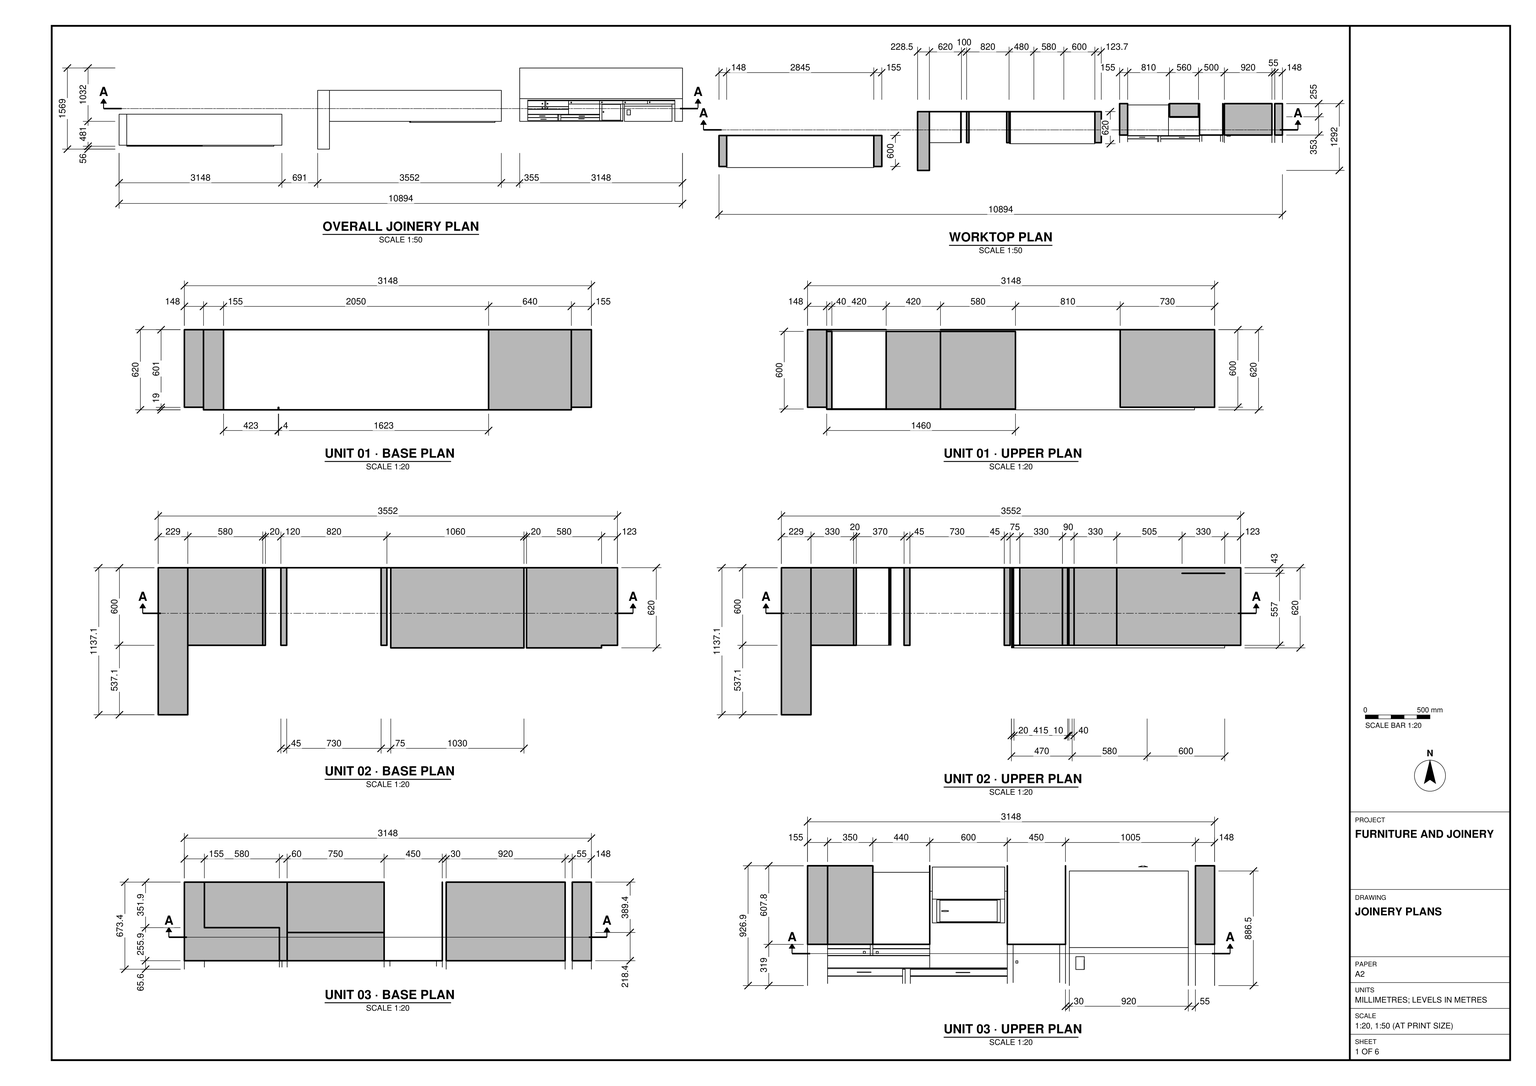
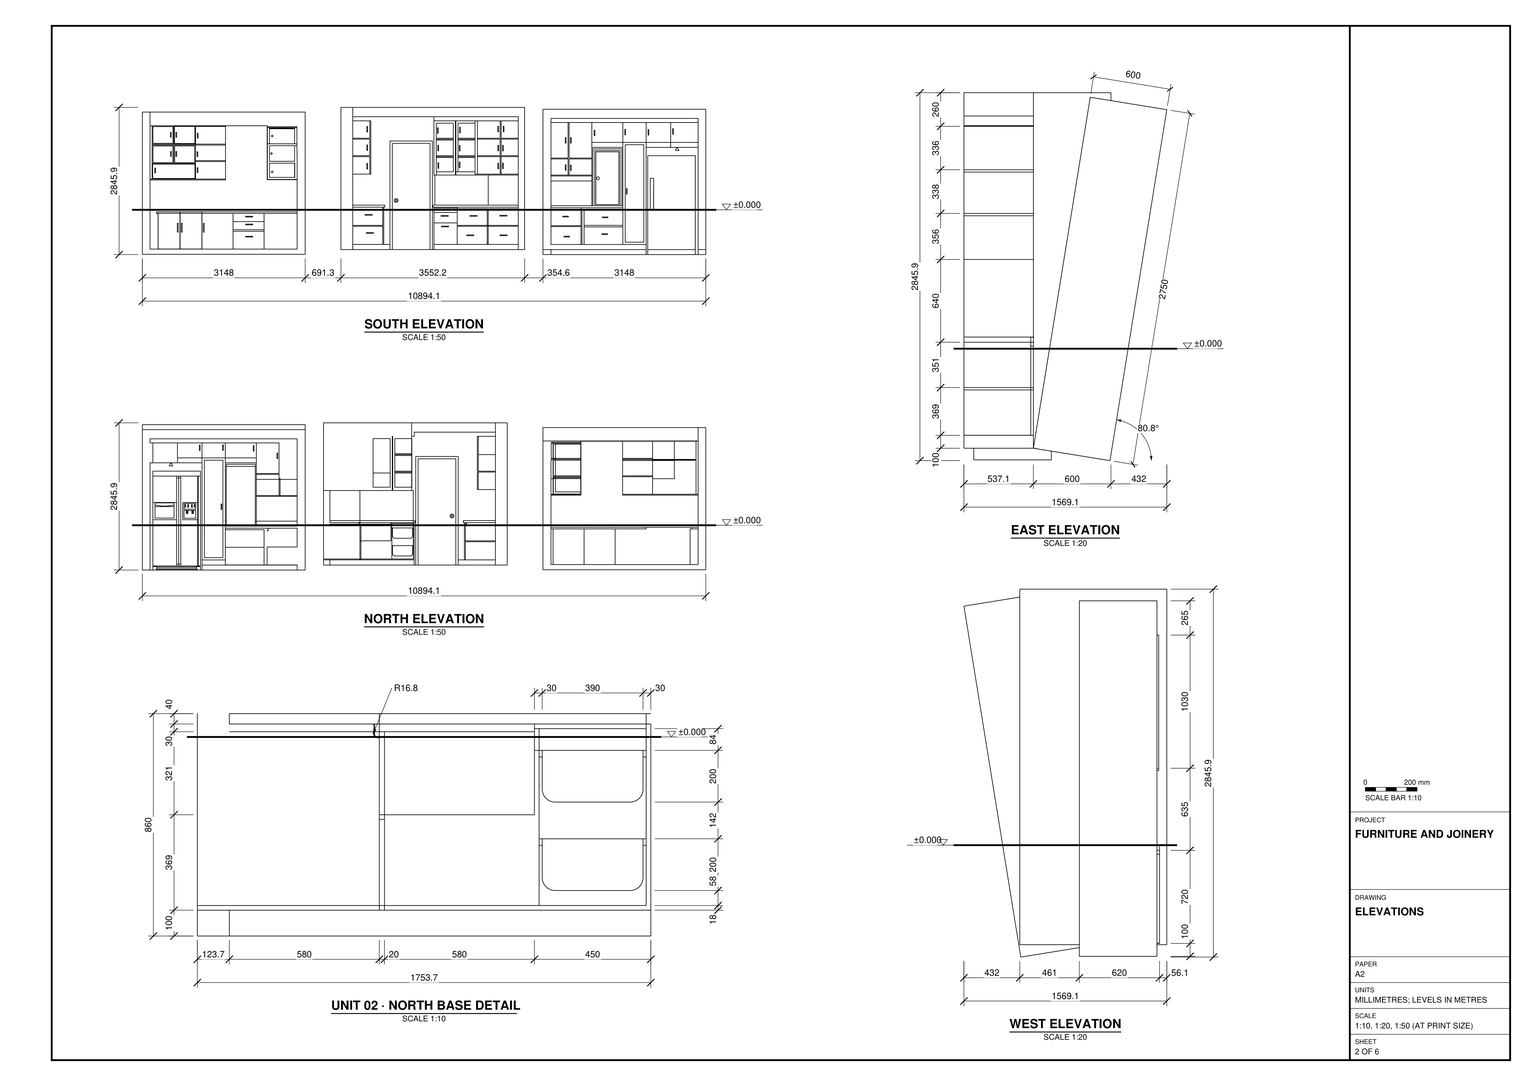
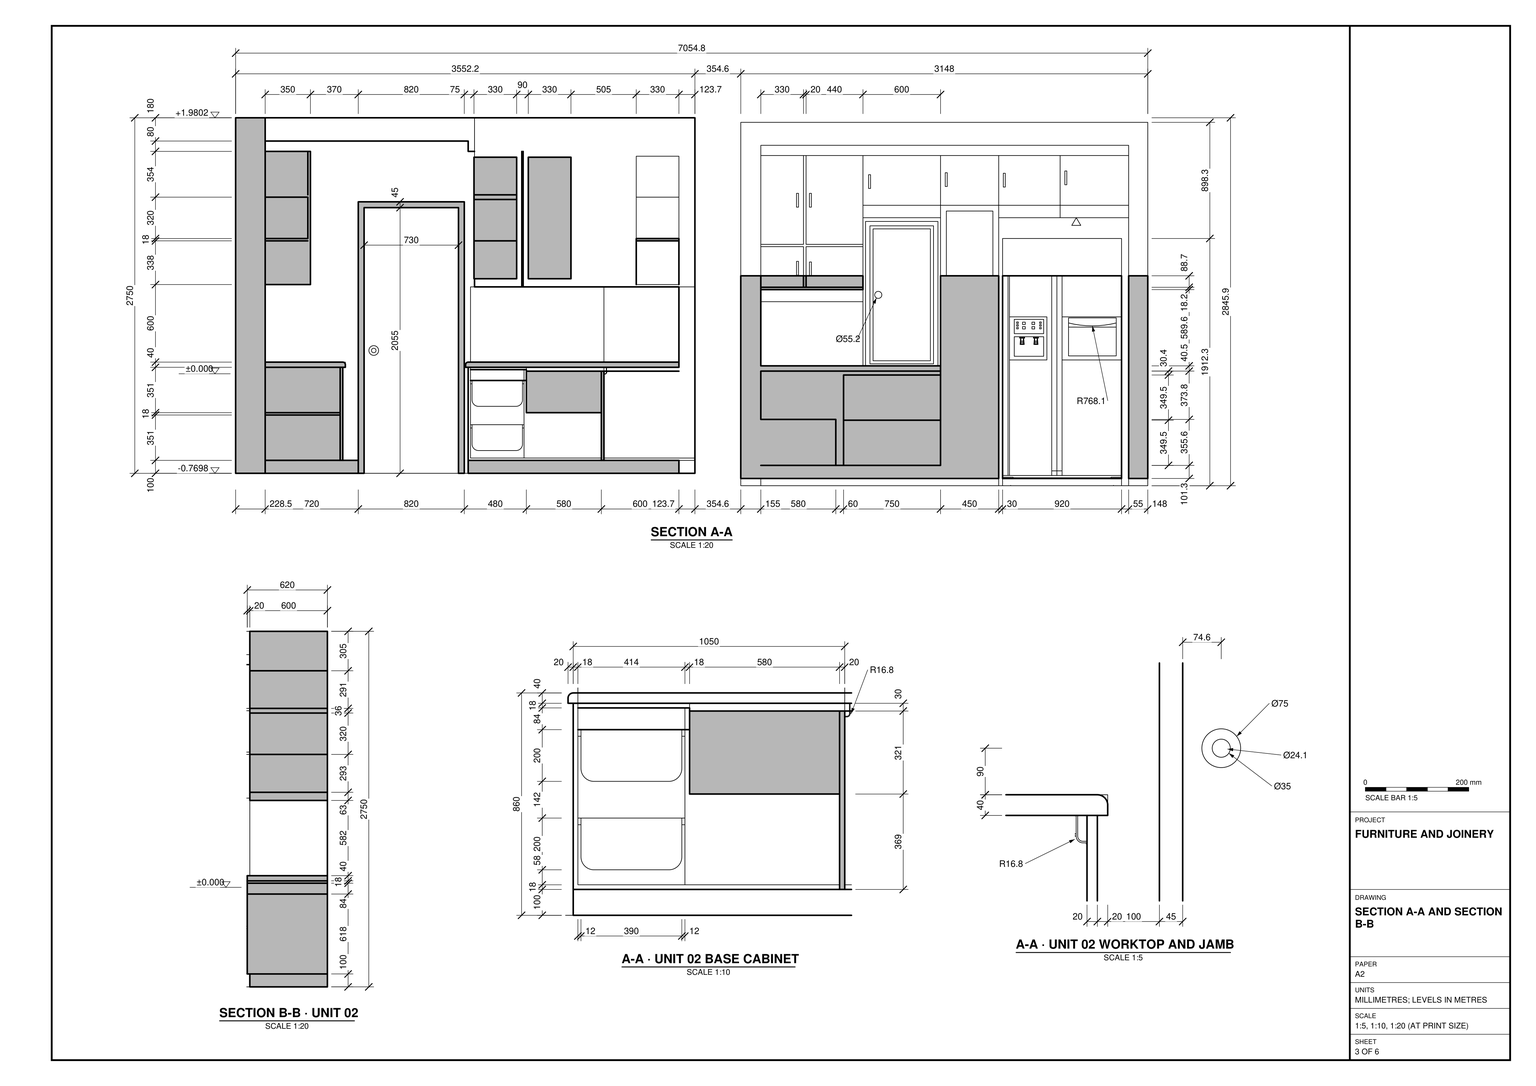
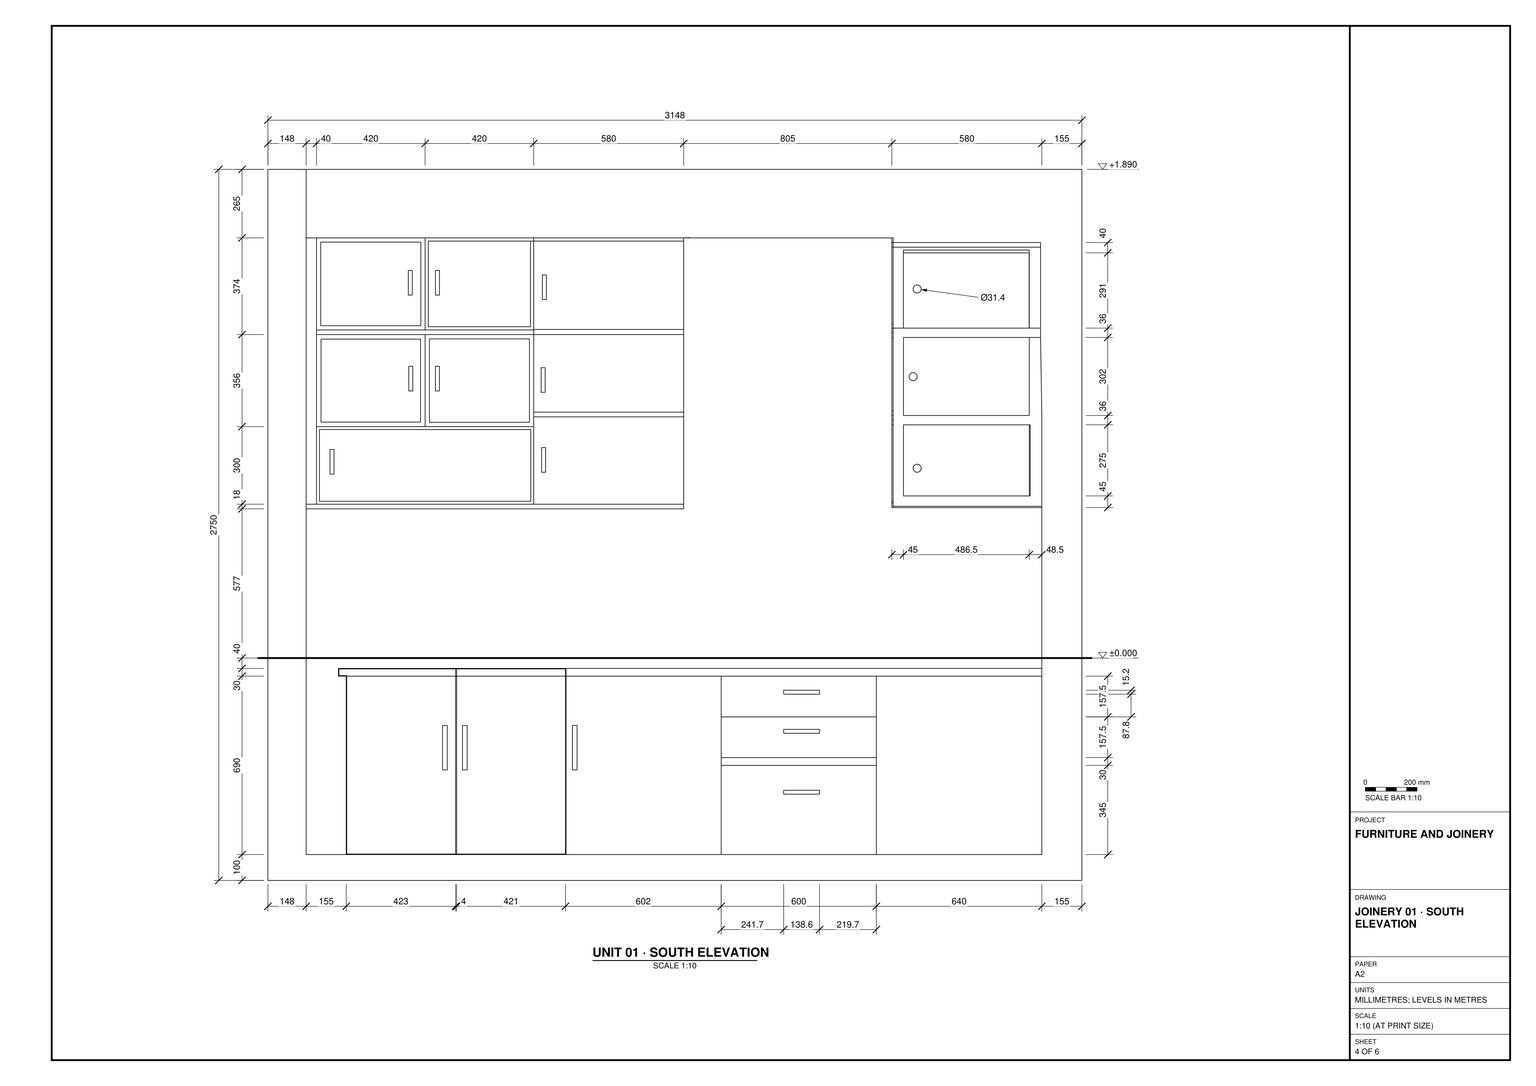
Build the three kitchen joinery runs in SketchUp from task_files/diagram_01.pdf. Work in millimetres. The complete arrangement is 10894.1 mm long, 1569.1 mm deep and 2845.9 mm high. Use the 0 mm reference level marked in the elevations; it crosses the joinery near the worktops, not at the plinths.

Use the overall plan to set out the gaps and front-to-back offsets between runs. Reading the south elevation from left to right, model the first run with base cupboards, drawers and two banks of upper cabinets separated by an open space. In the middle run, form the projecting end return and framed doorway, with worktops and storage to either side. Use the sections to model the plinths, worktop edges, shelves and stacked pull-outs at their drawn thicknesses. In the right-hand run, fit the base drawers, tall cabinet, refrigerator bay and overhead cupboards within the surround. Match the inclined and upright profiles shown together in the end elevations.

Appliances and any decorative or loose items shown may be suitable library components placed in the indicated positions. Keep each joinery assembly as a separate group or component and use components for repeated parts. Save one SketchUp model as output_files/three_kitchen_joinery_runs.skp.

# SketchUp Ruby script. Lengths in millimetres.
U = 1.mm
M = Sketchup.active_model
def pt(a) = Geom::Point3d.new(a.map { |v| v * U })
def face(e, loops, mat)
  f = e.add_face(loops[0].map { |a| pt(a) })
  loops[1..].each { |l| e.add_face(l.map { |a| pt(a) }).erase! }
  f.material = f.back_material = mat if mat
  f
end
# faces: each face lists its corners as indices into pts; further lists are holes
def faces(e, pts, list, mat = nil) = list.each { |f| face(e, (f[0].is_a?(Array) ? f : [f]).map { |l| l.map { |i| pts[i] } }, mat) }
# xy, xz, yz: faces in a plane at the given z, y or x. An outline is a flat list of corners, or four numbers for a rectangle; further outlines are holes
def ring(l) = l.size == 4 ? [[l[0], l[1]], [l[2], l[1]], [l[2], l[3]], [l[0], l[3]]] : l.each_slice(2).to_a
def flat(e, list, mat, &to3) = list.each { |f| face(e, (f[0].is_a?(Array) ? f : [f]).map { |l| ring(l).map { |u, v| to3.(u, v) } }, mat) }
def xy(e, z, list, mat = nil) = flat(e, list, mat) { |x, y| [x, y, z] }
def xz(e, y, list, mat = nil) = flat(e, list, mat) { |x, z| [x, y, z] }
def yz(e, x, list, mat = nil) = flat(e, list, mat) { |y, z| [x, y, z] }
def lines(e, pts, list) = list.each { |a, b| e.add_line(pt(pts[a]), pt(pts[b])) }
# prism: a flat outline (further loops are holes) pulled along v
def prism(e, loops, v, mat = nil)
  f = face(e, loops, mat); d = Geom::Vector3d.new(v.map { |x| x * U })
  f.pushpull(f.normal.samedirection?(d) ? d.length : -d.length)
end
def box(e, o, s, mat = nil) = prism(e, [[o, [o[0] + s[0], o[1], o[2]], [o[0] + s[0], o[1] + s[1], o[2]], [o[0], o[1] + s[1], o[2]]]], [0, 0, s[2]], mat)
def at(x, y, z, deg = 0) = Geom::Transformation.translation(pt([x, y, z])) * Geom::Transformation.rotation(ORIGIN, Z_AXIS, deg.degrees)
def axes(o, x, y, z) = Geom::Transformation.new([*x, 0, *y, 0, *z, 0, *pt(o).to_a, 1])
def part(name) = M.definitions.add(name)
# library, detail: a bought-in or finely detailed component or shape, given as its bounding box
def library(name, o, s) = part(name).tap { |d| box(d.entities, o, s) }
def detail(e, o, s) = box(e.add_group.entities, o, s)
def put(e, d, t, mat = nil) = e.add_instance(d, t).tap { |i| i.material = mat if mat }
def group(e, t, mat = nil) = e.add_group.tap { |g| g.transformation = t; g.material = mat if mat }.entities
root = M.entities
M.materials.add("A02_Rose_Quartz").color = [255, 153, 153]
M.materials.add("Asphalt_06_1K").color = [164, 157, 139]
M.materials.add("Denim_03_1K").color = [93, 106, 119]
M.materials.add("Glass_Basic_01").color = [161, 173, 186]
M.materials["Glass_Basic_01"].alpha = 0.2
M.materials.add("Glass_Safety_01").color = [204, 235, 244]
M.materials["Glass_Safety_01"].alpha = 0.2
M.materials.add("M09_Shadow_Night").color = [0, 0, 0]
M.materials.add("Wood_Floor_12_1K").color = [92, 75, 65]
M.materials.add("Wood_Veneer_15_1K").color = [103, 69, 45]
M.materials.add("glass").color = [0, 0, 0]
M.materials.add("white").color = [0, 0, 0]
c1 = library("fgkjh",[-49,-117.2,0],[98,234.4,0.1])
c2 = library("fkgjdg",[-460,-920,0],[920,1840,0.1])
c3 = part("sgdg")
p = [[83.1,0,0],[-83.1,-96,0],[-83.1,96,0]]
lines(c3.entities,p,[[0,1],[1,2],[2,0]])
c4 = library("Group\#26",[0,0,0],[920,1840,600])
c5 = part("fgklj")
p = [[-145,-100,0],[145,-100,0],[148.3,-99.9,0],[151.5,-99.6,0],[154.8,-99,0],[157.9,-98.3,0],
  [161.1,-97.3,0],[164.1,-96.2,0],[167.1,-94.8,0],[170,-93.3,0],[172.8,-91.6,0],[175.4,-89.7,0],
  [178,-87.6,0],[180.4,-85.4,0],[182.6,-83,0],[184.7,-80.4,0],[186.6,-77.8,0],[188.3,-75,0],
  [189.8,-72.1,0],[191.2,-69.1,0],[192.3,-66.1,0],[193.3,-62.9,0],[194,-59.8,0],[194.6,-56.5,0],
  [194.9,-53.3,0],[195,-50,0],[195,100,0],[-195,100,0],[-195,-50,0],[-194.9,-53.3,0],
  [-194.6,-56.5,0],[-194,-59.8,0],[-193.3,-62.9,0],[-192.3,-66.1,0],[-191.2,-69.1,0],[-189.8,-72.1,0],
  [-188.3,-75,0],[-186.6,-77.8,0],[-184.7,-80.4,0],[-182.6,-83,0],[-180.4,-85.4,0],[-178,-87.6,0],
  [-175.4,-89.7,0],[-172.8,-91.6,0],[-170,-93.3,0],[-167.1,-94.8,0],[-164.1,-96.2,0],[-161.1,-97.3,0],
  [-157.9,-98.3,0],[-154.8,-99,0],[-151.5,-99.6,0],[-148.3,-99.9,0],[-207,100,0],[-207,74.5,0],
  [-195,74.5,0],[207,100,0],[207,74.5,0],[195,74.5,0]]
lines(c5.entities,p,[[0,1],[1,2],[2,3],[3,4],[4,5],[5,6],[6,7],[7,8],[8,9],[9,10],[10,11],[11,12],
  [12,13],[13,14],[14,15],[15,16],[16,17],[17,18],[18,19],[19,20],[20,21],[21,22],[22,23],[23,24],
  [24,25],[25,26],[26,27],[27,28],[28,29],[29,30],[30,31],[31,32],[32,33],[33,34],[34,35],[35,36],
  [36,37],[37,38],[38,39],[39,40],[40,41],[41,42],[42,43],[43,44],[44,45],[45,46],[46,47],[47,48],
  [48,49],[49,50],[50,51],[51,0],[27,52],[52,53],[53,54],[54,27],[26,55],[55,56],[56,57],[57,26]])
g1 = group(root,at(7746.2,1129.4,-350.7))
yz(g1,0,[[0,0,-592.3,95.9,-152.6,2810.6,439.7,2714.6]])
yz(g1,155,[[72.1,445.2,75,463,-517.3,558.9,-520.2,541.1],[137.5,848.9,230.5,1423.5,-361.7,1519.4,-454.8,944.9]])
yz(g1,155,[[75,463,-517.3,558.9,-461.2,905.4,131.1,809.5],[230.5,1423.5,-361.7,1519.4,-358.9,1537.1,233.4,1441.2],[233.4,1441.2,-358.9,1537.1,-308.3,1849.1,283.9,1753.2],[283.9,1753.2,-308.3,1849.1,-305.5,1866.9,286.8,1770.9],[286.8,1770.9,-305.5,1866.9,-194.2,2553.9,398.1,2458],
  [398.1,2458,-194.2,2553.9,-181.4,2632.9,410.9,2536.9]],"Wood_Floor_12_1K")
yz(g1,485,[[233.4,1441.2,283.9,1753.2,-308.3,1849.1,-358.9,1537.1]])
yz(g1,505,[[233.4,1441.2,283.9,1753.2,-308.3,1849.1,-358.9,1537.1],[286.8,1770.9,398.1,2458,-194.2,2553.9,-305.5,1866.9]])
yz(g1,735,[[16,98.7,-576.3,194.6,-520.2,541.1,72.1,445.2]])
yz(g1,795,[[16,98.7,71.1,439.3,-521.1,535.2,-576.3,194.6],[71.1,439.3,75.9,468.9,-516.3,564.8,-521.1,535.2],[75.9,468.9,126.3,779.8,-466,875.8,-516.3,564.8]])
yz(g1,945,[[230.5,1423.5,-361.7,1519.4,-358.9,1537.1,233.4,1441.2],[233.4,1441.2,283.9,1753.2,-308.3,1849.1,-358.9,1537.1],[283.9,1753.2,286.8,1770.9,-305.5,1866.9,-308.3,1849.1],[286.8,1770.9,-305.5,1866.9,-256.5,2168.9,335.8,2073]],"Wood_Floor_12_1K")
yz(g1,965,[[140.7,868.7,-107.4,908.9,76.5,2044.1,324.6,2003.9]])
yz(g1,1525,[[140.7,868.7,324.6,2003.9,76.5,2044.1,-107.4,908.9]])
yz(g1,1545,[[16,98.7,71.1,439.3,-521.1,535.2,-576.3,194.6],[71.1,439.3,75.9,468.9,-516.3,564.8,-521.1,535.2],[75.9,468.9,126.3,779.8,-466,875.8,-516.3,564.8],[126.3,779.8,131.1,809.5,-461.2,905.4,-466,875.8],[131.1,809.5,137.5,848.9,-454.8,944.9,-461.2,905.4]])
yz(g1,1545,[[137.5,848.9,-454.8,944.9,-256.5,2168.9,335.8,2073]],"Wood_Floor_12_1K")
yz(g1,1995,[[0,0,16,98.7,-576.3,194.6,-592.3,95.9],[16,98.7,335.8,2073,-256.5,2168.9,-576.3,194.6]],"Wood_Floor_12_1K")
yz(g1,3000,[[0,0,-592.3,95.9,-256.5,2168.9,335.8,2073],[398.1,2458,410.9,2536.9,-181.4,2632.9,-194.2,2553.9]],"Wood_Floor_12_1K")
yz(g1,3148,[[0,0,439.7,2714.6,-152.6,2810.6,-592.3,95.9]])
# 9 loose lines left out
p = [[0,0,0],[155,0,0],[155,-592.3,95.9],[0,-592.3,95.9],[1995,0,0],[1995,-592.3,95.9],
  [3000,0,0],[3148,0,0],[3148,-592.3,95.9],[3000,-592.3,95.9],[3000,398.1,2458],[2945,398.1,2458],
  [2945,335.8,2073],[3000,335.8,2073],[3148,439.7,2714.6],[0,439.7,2714.6],[155,16,98.7],[735,16,98.7],
  [735,72.1,445.2],[155,72.1,445.2],[155,75,463],[155,131.1,809.5],[735,131.1,809.5],[1545,131.1,809.5],
  [1545,137.5,848.9],[945,137.5,848.9],[155,137.5,848.9],[155,230.5,1423.5],[155,233.4,1441.2],[155,283.9,1753.2],
  [155,286.8,1770.9],[155,398.1,2458],[155,410.9,2536.9],[3000,410.9,2536.9],[2025,294.2,1816.3],[2025,0,0],
  [2945,0,0],[2945,294.2,1816.3],[735,-576.3,194.6],[155,-576.3,194.6],[155,-520.2,541.1],[155,-517.3,558.9],
  [155,-461.2,905.4],[155,-454.8,944.9],[155,-361.7,1519.4],[155,-358.9,1537.1],[155,-308.3,1849.1],[155,-305.5,1866.9],
  [155,-194.2,2553.9],[155,-181.4,2632.9],[3000,-181.4,2632.9],[3000,-194.2,2553.9],[3000,-256.5,2168.9],[3148,-152.6,2810.6],
  [0,-152.6,2810.6],[1995,-576.3,194.6],[1545,-576.3,194.6],[795,-576.3,194.6],[755,-576.3,194.6],[755,16,98.7],
  [795,16,98.7],[1545,16,98.7],[795,71.1,439.3],[795,75.9,468.9],[795,126.3,779.8],[1545,126.3,779.8],
  [1545,71.1,439.3],[735,-520.2,541.1],[513.8,-550.2,355.5],[513.8,-552.7,340.5],[405.7,-552.7,340.5],[405.7,-550.2,355.5],
  [735,-461.2,905.4],[735,-466,875.8],[755,-466,875.8],[795,-521.1,535.2],[795,-516.3,564.8],[795,-466,875.8],
  [1545,-466,875.8],[1545,-461.2,905.4],[735,-517.3,558.9],[1545,-521.1,535.2],[1140.1,-542.6,402.6],[1248.3,-542.6,402.6],
  [1248.3,-545,387.6],[1140.1,-545,387.6],[1995,-256.5,2168.9],[1545,-256.5,2168.9],[1545,-454.8,944.9],[1545,-516.3,564.8],
  [1950,-569.1,239.1],[1590,-569.1,239.1],[1590,-263.7,2124.5],[1950,-263.7,2124.5],[1626.5,-401,1277],[1626.5,-418.3,1170.3],
  [1611.3,-418.3,1170.3],[1611.3,-401,1277],[1545,75.9,468.9],[491.3,-487.5,742.8],[491.3,-490,727.7],[383.2,-490,727.7],
  [383.2,-487.5,742.8],[1255.6,-490,727.3],[1255.6,-492.5,712.2],[1147.5,-492.5,712.2],[1147.5,-490,727.3],[945,-454.8,944.9],
  [965,140.7,868.7],[1525,140.7,868.7],[1525,-107.4,908.9],[965,-107.4,908.9],[965,324.6,2003.9],[1525,324.6,2003.9],
  [1525,76.5,2044.1],[965,76.5,2044.1],[999.2,-101.9,942.6],[999.2,71,2010.3],[1490.8,71,2010.3],[1490.8,-101.9,942.6],
  [1023.3,-98,966.4],[1023.3,67.2,1986.5],[1466.7,67.2,1986.5],[1466.7,-98,966.4],[1082.9,-18.7,1456.6],[1077.1,-19.4,1452.3],
  [1070.4,-19.8,1449.5],[1063.2,-20,1448.6],[1056,-19.8,1449.6],[1049.3,-19.3,1452.3],[1043.6,-18.6,1456.7],[1039.2,-17.7,1462.4],
  [1036.5,-16.6,1469],[1035.5,-15.5,1476.1],[1036.5,-14.3,1483.2],[1039.3,-13.3,1489.8],[1043.7,-12.4,1495.5],[1049.5,-11.7,1499.9],
  [1056.2,-11.2,1502.6],[1063.4,-11.1,1503.5],[1070.6,-11.2,1502.5],[1077.3,-11.7,1499.8],[1083,-12.4,1495.4],[1087.4,-13.3,1489.7],
  [1090.2,-14.4,1483.1],[1091.1,-15.5,1476],[1090.1,-16.7,1468.9],[1087.3,-17.7,1462.3],[230,230.5,1423.5],[945,230.5,1423.5],
  [945,-361.7,1519.4],[230,233.4,1441.2],[230,-358.9,1537.1],[485,233.4,1441.2],[485,-358.9,1537.1],[505,233.4,1441.2],
  [505,-358.9,1537.1],[945,233.4,1441.2],[945,-358.9,1537.1],[485,283.9,1753.2],[505,283.9,1753.2],[945,283.9,1753.2],
  [485,-194.2,2553.9],[485,-305.5,1866.9],[485,-308.3,1849.1],[505,-308.3,1849.1],[945,-308.3,1849.1],[945,-305.5,1866.9],
  [505,-305.5,1866.9],[505,-194.2,2553.9],[446.5,-326.8,1735.4],[446.5,-344,1628.6],[431.2,-344,1628.6],[431.2,-326.8,1735.4],
  [546.4,-327.5,1730.6],[546.4,-344.8,1623.8],[531.1,-344.8,1623.8],[531.1,-327.5,1730.6],[505,398.1,2458],[505,286.8,1770.9],
  [485,286.8,1770.9],[2470,398.1,2458],[1995,398.1,2458],[1545,398.1,2458],[945,398.1,2458],[446.5,-241.6,2261.3],
  [446.5,-258.9,2154.5],[431.2,-258.9,2154.5],[431.2,-241.6,2261.3],[945,-194.2,2553.9],[945,-256.5,2168.9],[546.4,-258.9,2154.5],
  [546.4,-241.6,2261.3],[531.1,-241.6,2261.3],[531.1,-258.9,2154.5],[1545,335.8,2073],[945,335.8,2073],[2470,335.8,2073],
  [1995,335.8,2073],[2470,-256.5,2168.9],[1545,-194.2,2553.9],[1003.9,-235.5,2299],[1003.9,-218.2,2405.8],[988.6,-218.2,2405.8],
  [988.6,-235.5,2299],[1995,-194.2,2553.9],[1596.9,-233,2314.3],[1596.9,-215.7,2421.1],[1581.7,-215.7,2421.1],[1581.7,-233,2314.3],
  [2470,-194.2,2553.9],[2045.8,-233.7,2310],[2045.8,-216.4,2416.8],[2030.6,-216.4,2416.8],[2030.6,-233.7,2310],[2945,-194.2,2553.9],
  [2521.7,-213.5,2434.6],[2521.7,-230.8,2327.8],[2506.5,-230.8,2327.8],[2506.5,-213.5,2434.6]]
faces(g1,p,[[0,1,2,3],[1,4,5,2],[6,7,8,9],[38,39,40,41,42,43,44,45,46,47,48,49,50,51,52,9,8,53,54,3,2,5,55,56,57,58],[16,17,38,39],[[38,67,40,39],[68,69,70,71]],[[81,75,57,56],[82,83,84,85]],[[91,90,93,92],[94,95,96,97]],
  [[72,42,41,80,73],[99,100,101,102]],[[78,77,76,89],[103,104,105,106]],[27,148,149,150,44],[151,148,27,28],[45,44,150,158,156,154,152],[[154,164,46,45,152],[170,171,172,173]],[[158,166,165,156],[174,175,176,177]],[[163,162,48,47],[185,186,187,188]],
  [[167,168,169,189,190],[191,192,193,194]],[195,196,190,87],[197,198,86,199],[13,52,199,197,12],[[200,87,190,189],[201,202,203,204]],[[87,200,205,86],[206,207,208,209]],[[199,86,205,210],[211,212,213,214]],[[199,52,51,215,210],[216,217,218,219]],
  [33,32,49,50],[162,169,189,200,205,210,215,51,50,49,48]],"Wood_Floor_12_1K")
faces(g1,p,[[10,11,12,13,6,7,14,15,0,1,16,17,18,19,20,21,22,23,24,25,26,27,28,29,30,31,32,33],[34,35,36,37],[59,60,57,58],[61,60,57,56],[18,17,59,60,62,63,64,65,23,22,21,20,19],[62,66,61,60],[66,62,75,81],[66,98,65,64,63,62],
  [19,18,67,40],[64,65,78,77],[22,21,42,72],[23,22,72,79],[25,26,43,107],[24,25,107,88],[108,109,110,111],[112,113,109,108],
  [45,152,151,28],[153,151,152,154],[155,156,154,153],[155,157,158,156],[159,153,151,28,29],[160,155,153,159],[160,161,157,155],[29,159,164,46],
  [161,160,165,166],[178,179,180,159,29,30,31,32,33,10,11,181,182,183,184],[159,180,179,160],[113,112,115,114],[197,12,11,181],[178,184,189,169],[184,183,200,189],[183,182,205,200],
  [182,181,210,205],[11,181,210,215],[51,10,11,215],[14,15,54,53]])
faces(g1,p,[[17,59,58,38],[72,73,74,58,57,75,76,77,78,79],[73,80,67,38,58,74],[[56,55,86,87,88,79,78,89,81],[90,91,92,93]],[89,76,75,81],[80,41,40,67],[42,72,79,88,107,43],[125,124,147,146,145,144,143,142,141,140,139,138,137,136,135,134,133,132,131,130,129,128,127,126],
  [162,163,47,46,164,154,156,165,166,167,168,169]],"M09_Shadow_Night")
faces(g1,p,[[69,68,71,70],[84,83,82,85],[104,103,106,105],[100,99,102,101],[96,95,94,97],[176,175,174,177],[172,171,170,173],[187,186,185,188],
  [194,191,192,193],[204,201,202,203],[214,211,212,213],[209,206,207,208],[218,217,216,219]],"glass")
faces(g1,p,[[[114,115,111,110],[116,117,118,119]],[[117,116,119,118],[120,121,122,123]],[[121,120,123,122],[124,125,126,127,128,129,130,131,132,133,134,135,136,137,138,139,140,141,142,143,144,145,146,147]]],"A02_Rose_Quartz")
put(g1,c1,axes([723.5,126.7,782.3],[-0.23471,0,0],[0,0.03753,0.23169],[0,-0.23169,0.03753]))
put(g1,c2,axes([2485,147.1,908.2],[1,0,0],[0,0.15988,0.98714],[0,-0.98714,0.15988]))
put(g1,c3,axes([2594.9,330.9,2043.1],[0,0.05813,0.35888],[-0.36355,0,0],[0,-0.35888,0.05813]))
put(g1,c4,axes([2025,0,0],[1,0,0],[0,0.15988,0.98714],[0,-0.98714,0.15988]),"Denim_03_1K")
g2 = group(root,at(3839.3,1137.1,-254.8))
xy(g2,0,[[0,-1137.1,228.5,0]])
xy(g2,0,[[228.5,-600,948.5,0],[3428.5,-600,3552.2,0]],"Wood_Floor_12_1K")
xy(g2,100,[[1798.5,-620,2248.5,0],[2848.5,-620,3428.5,0]])
xy(g2,100.5,[[228.5,-600,808.5,0]])
xy(g2,451,[[228.5,-600,808.5,0]])
xy(g2,469,[[2248.5,-620,2828.5,0],[228.5,-600,808.5,0]])
xy(g2,718,[[1816.5,-620,2248.5,0]])
xy(g2,790,[[2248.5,-620,2828.5,0],[2828.5,-620,2848.5,0],[2848.5,-620,3428.5,0]])
xy(g2,802,[[1816.5,-620,2248.5,0]])
xy(g2,820,[[1798.5,-620,1816.5,0],[1816.5,-620,2248.5,0],[2248.5,-620,3428.5,0],[228.5,-600,808.5,0]])
xy(g2,1442,[[2213.5,-600,2223.5,0]])
xy(g2,1442,[[1847.6,-600,2213.5,0],[2223.5,-600,2593.5,0],[2593.5,-600,3428.5,0]],"Wood_Floor_12_1K")
xy(g2,1460,[[228.5,-600,578.5,0]],"Wood_Floor_12_1K")
xy(g2,1505,[[2263.5,-600,2593.5,0]])
xy(g2,1505,[[1843.5,-600,1847.6,0],[1847.6,-600,2173.5,0]],"Wood_Floor_12_1K")
xy(g2,1798,[[228.5,-600,558.5,0],[1843.5,-600,2173.5,0],[3098.5,-600,3428.5,-43]])
xy(g2,1816,[[228.5,-600,558.5,0],[3098.5,-600,3428.5,-43]])
xy(g2,2118,[[1843.5,-600,2173.5,0]])
xy(g2,2136,[[228.5,-600,558.5,0]])
xy(g2,2154,[[1843.5,-600,2173.5,0]])
xy(g2,2445,[[1843.5,-600,1847.6,0],[1847.6,-600,2173.5,0],[2263.5,-600,2593.5,0]])
xy(g2,2490,[[228.5,-600,558.5,0],[558.5,-600,578.5,0],[1798.5,-600,1847.6,0]],"Wood_Floor_12_1K")
xy(g2,2570,[[228.5,-600,1798.5,0]],"Wood_Floor_12_1K")
xy(g2,2750,[[0,-1137.1,228.5,0]])
xy(g2,2750,[[228.5,-600,3552.2,0]],"Wood_Floor_12_1K")
xz(g2,-1137.1,[[0,0,228.5,2750]])
xz(g2,-620,[[2248.5,451,2828.5,469],[2848.5,451,3428.5,469],[2248.5,790,3428.5,820],[1798.5,802,2248.5,820]],"M09_Shadow_Night")
xz(g2,-620,[[[2248.5,100,2828.5,451],[2432.3,269.3,2571,284.6]],[[2848.5,100,3428.5,451],[3075.8,269.3,3214.5,284.6]],[[2848.5,469,3428.5,790],[3072.9,648.2,3211.5,663.5]],[[1798.5,516.6,2248.5,718],[1936.4,644.4,2075.1,659.7]],[1798.5,718,2248.5,802]],"Wood_Floor_12_1K")
xz(g2,-620,[[[1798.5,100,2248.5,516.6],[1943.7,439.1,2082.4,454.4]],[2432.3,269.3,2571,284.6],[3075.8,269.3,3214.5,284.6],[1943.7,439.1,2082.4,454.4],[1936.4,644.4,2075.1,659.7],
  [2493.8,644.4,2632.4,659.7],[3072.9,648.2,3211.5,663.5]],"glass")
xz(g2,-600,[[228.5,100,828.5,100,828.5,100.4]])
xz(g2,-600,[[228.5,451,808.5,469],[1798.5,1442,1798.5,2490,2213.5,2490,2213.5,1442,1847.6,1442,1847.6,1505,2173.5,1505,2173.5,2445,1843.5,2445,1843.5,1505,1847.6,1505,1847.6,1442],[2213.5,1442,2223.5,2490],[2223.5,1442,2593.5,1505],[2593.5,1442,3428.5,1460],
  [558.5,1460,578.5,1460,578.5,2490,558.5,2490,558.5,2154,228.5,2154,228.5,2136,558.5,2136,558.5,1816,228.5,1816,228.5,1798,558.5,1798],[2593.5,1460,2638.5,2490],[3078.5,1460,3098.5,2136],[2223.5,1505,2223.5,2490,2593.5,2490,2593.5,2445,2263.5,2445,2263.5,1505],[1843.5,1780,2173.5,1798],
  [2263.5,1780,2593.5,1798],[1843.5,1798,2173.5,1816],[2263.5,1798,2593.5,1816],[2638.5,1798,3078.5,1816],[3098.5,1798,3428.5,1816],
  [1843.5,2118,2173.5,2136],[2263.5,2118,2593.5,2136],[1843.5,2136,2173.5,2154],[2263.5,2136,2593.5,2154],[2638.5,2136,3428.5,2136,3428.5,2154,3098.5,2154,3098.5,2490,3078.5,2490,3078.5,2154,2638.5,2154]],"M09_Shadow_Night")
xz(g2,-600,[[228.5,0,948.5,0,948.5,100.5,828.5,100.4,828.5,100,228.5,100],[3428.5,0,3552.2,0,3552.2,2750,228.5,2750,228.5,2570,3428.5,2570],[[228.5,100.5,808.5,451],[490.7,314.7,629.3,330]],[[228.5,469,808.5,820],[466.5,664.8,605.2,680]],[[228.5,1460,558.5,1798],[500.3,1558.2,515.5,1666.4]],
  [[2638.5,1460,3078.5,1798],[3033.7,1562.9,3049,1671.1]],[[3098.5,1460,3428.5,1798],[3125,1565.2,3140.3,1673.4]],[[1843.5,1505,2173.5,1780],[1875.4,1571.3,1890.6,1679.4]],[[2263.5,1505,2593.5,1780],[2287.5,1585.3,2302.7,1693.4]],[[228.5,1816,558.5,2136],[501.6,1916.7,516.8,2024.8]],
  [[1843.5,1816,2173.5,2118],[1873.4,1909.2,1888.7,2017.3]],[[2263.5,1816,2593.5,2118],[2288.1,1906.8,2303.4,2015]],[[2638.5,1816,3078.5,2136],[3034.4,1908.7,3049.7,2016.9]],[[3098.5,1816,3428.5,2136],[3125.3,1908.2,3140.5,2016.4]],[[228.5,2154,558.5,2490],[501.2,2274,516.5,2382.2]],
  [[1843.5,2154,2173.5,2445],[1865.8,2248.4,1881,2356.5]],[[2263.5,2154,2593.5,2445],[2292.9,2258.3,2308.1,2366.5]],[[2638.5,2154,3078.5,2490],[3032.6,2277,3047.8,2385.2]],[[3098.5,2154,3428.5,2490],[3138,2277,3153.2,2385.2]],[1798.5,2490,3428.5,2570]],"Wood_Floor_12_1K")
xz(g2,-600,[[490.7,314.7,629.3,330],[466.5,664.8,605.2,680],[500.3,1558.2,515.5,1666.4],[3033.7,1562.9,3049,1671.1],[3125,1565.2,3140.3,1673.4],
  [1875.4,1571.3,1890.6,1679.4],[2287.5,1585.3,2302.7,1693.4],[2288.1,1906.8,2303.4,2015],[3125.3,1908.2,3140.5,2016.4],[3034.4,1908.7,3049.7,2016.9],
  [1873.4,1909.2,1888.7,2017.3],[501.6,1916.7,516.8,2024.8],[1865.8,2248.4,1881,2356.5],[2292.9,2258.3,2308.1,2366.5],[501.2,2274,516.5,2382.2],
  [3032.6,2277,3047.8,2385.2],[3138,2277,3153.2,2385.2]],"glass")
xz(g2,-43,[[3098.5,1460,3428.5,1798],[3098.5,1798,3428.5,1816],[3098.5,1816,3428.5,2136],[3098.5,2136,3428.5,2452.6]])
xz(g2,0,[[0,0,228.5,2750],[228.5,0,228.5,100,828.5,100,828.5,100.4,948.5,100.5,948.5,0],[948.5,0,948.5,100.5,808.5,100.5,808.5,820,228.5,820,228.5,1460,578.5,1460,578.5,2490,228.5,2490,228.5,2570,1798.5,2570,1798.5,2490,1847.6,2490,1847.6,2445,1843.5,2445,1843.5,1505,1847.6,1505,1847.6,1442,1816.5,1442,1816.5,820,1798.5,820,1798.5,100,3428.5,100,3428.5,0],[3428.5,0,3552.2,100],[228.5,100,808.5,100,808.5,100.4],
  [228.5,100,808.5,100.4,228.5,100.4],[808.5,100,828.5,100.4],[1798.5,100,2828.5,100,2828.5,118,1816.5,118,1816.5,820,1798.5,820],[2828.5,100,2848.5,118],[2848.5,100,3552.2,118],
  [228.5,100.4,808.5,100.5],[808.5,100.4,828.5,100.5],[828.5,100.4,828.5,100.5,948.5,100.5],[228.5,100.5,808.5,451],[1816.5,118,2828.5,118,2828.5,469,2248.5,469,2248.5,718,1816.5,718],
  [2828.5,118,2848.5,451],[2848.5,118,3552.2,118,3552.2,1442,3428.5,1442,3428.5,820,2848.5,820],[228.5,451,808.5,469],[2828.5,451,2848.5,469],[228.5,469,808.5,820],
  [2828.5,469,2848.5,790],[1816.5,718,2248.5,802],[2248.5,790,2848.5,820],[1816.5,802,2248.5,820],[1816.5,820,2848.5,1442],
  [2848.5,820,3428.5,1442],[[1847.6,1442,1847.6,1505,2173.5,1505,2173.5,2445,1847.6,2445,1847.6,2750,3552.2,2750,3552.2,1442,2223.5,1442,2223.5,2490,2213.5,2490,2213.5,1442],[2263.5,1505,2593.5,2445]],[2213.5,1442,2223.5,2490],[228.5,1460,558.5,1798],[558.5,1460,578.5,2490],
  [1843.5,1505,1847.6,1780],[1847.6,1505,2173.5,1780],[2263.5,1505,2593.5,1780],[1843.5,1780,1847.6,1798],[1847.6,1780,2173.5,1798],
  [2263.5,1780,2593.5,2445],[228.5,1798,558.5,1816],[1843.5,1798,1847.6,1816],[1847.6,1798,2173.5,1816],[228.5,1816,558.5,2136],
  [1843.5,1816,1847.6,2118],[1847.6,1816,2173.5,2118],[1843.5,2118,1847.6,2136],[1847.6,2118,2173.5,2136],[228.5,2136,558.5,2490],
  [1843.5,2136,1847.6,2154],[1847.6,2136,2173.5,2154],[1843.5,2154,1847.6,2445],[1847.6,2154,2173.5,2445],[1798.5,2490,1798.5,2570,228.5,2570,228.5,2750,1847.6,2750,1847.6,2490]])
yz(g2,0,[[-1137.1,0,0,2750]])
yz(g2,228.5,[[-1137.1,0,-600,100],[-600,0,0,100],[-1137.1,100,0,100.4],[-1137.1,100.4,0,100.5],[-1137.1,100.5,-600,451],
  [-600,100.5,0,451],[-1137.1,451,-600,469],[-600,451,0,469],[-1137.1,469,-600,820],[-600,469,0,820],
  [-1137.1,820,0,860],[-1137.1,860,0,1460],[-1137.1,1460,-600,1798],[-600,1460,0,1798],[-1137.1,1798,-600,1816],
  [-600,1798,0,1816],[-1137.1,1816,-600,2136],[-600,1816,0,2136],[-1137.1,2136,-600,2154],[-600,2136,0,2154],
  [-1137.1,2154,-600,2490],[-600,2154,0,2490],[-1137.1,2490,0,2495],[-1137.1,2495,0,2570],[-1137.1,2570,-600,2750],
  [-600,2570,0,2750]])
yz(g2,558.5,[[-600,1816,0,2136],[-600,2154,0,2490]])
yz(g2,578.5,[[-600,1460,0,2490]],"Wood_Floor_12_1K")
yz(g2,808.5,[[-600,100.5,0,451],[-600,451,0,469],[-600,469,0,790],[-600,790,0,820]])
yz(g2,948.5,[[-600,0,0,100.5]])
yz(g2,1798.5,[[-620,100,0,820]])
yz(g2,1798.5,[[-600,2490,0,2570]],"Wood_Floor_12_1K")
yz(g2,1843.5,[[-600,1505,0,1780],[-600,1780,0,1798],[-600,1798,0,1816],[-600,1816,0,2118],[-600,2118,0,2136],
  [-600,2136,0,2154],[-600,2154,0,2445]],"Wood_Floor_12_1K")
yz(g2,1847.6,[[-600,1442,0,1505]])
yz(g2,2173.5,[[-600,1505,0,1780],[-600,1780,0,1798],[-600,1798,0,1816],[-600,1816,0,2118],[-600,2118,0,2136],
  [-600,2136,0,2154],[-600,2154,0,2445]])
yz(g2,2213.5,[[-600,1442,0,1780],[-600,1780,0,2467],[-600,2467,0,2490]])
yz(g2,2223.5,[[-600,1442,0,1505],[-600,1505,0,1780],[-600,1780,0,2467],[-600,2467,0,2490]])
yz(g2,2248.5,[[-620,469,0,516.6],[-620,516.6,0,718],[-620,718,0,790],[-620,790,0,802]])
yz(g2,2263.5,[[-600,1505,0,1780],[-600,1780,0,1798],[-600,1798,0,1816],[-600,1816,0,2118],[-600,2118,0,2136],
  [-600,2136,0,2154],[-600,2154,0,2445]])
yz(g2,2593.5,[[-600,1505,0,1780],[-600,1780,0,1798],[-600,1798,0,1816],[-600,1816,0,2118],[-600,2118,0,2136],
  [-600,2136,0,2154],[-600,2154,0,2445]])
yz(g2,2828.5,[[-620,100,0,451],[-620,451,0,469]],"Wood_Floor_12_1K")
yz(g2,2848.5,[[-620,100,0,451],[-620,451,0,469],[-620,469,0,790]],"Wood_Floor_12_1K")
yz(g2,3098.5,[[-600,1460,-43,1798],[-600,1798,-43,1816]])
yz(g2,3428.5,[[-600,0,0,100],[-620,100,-600,451],[-620,451,-600,469],[-620,469,-600,790],[-620,790,-600,820],
  [-600,820,0,860],[-600,1460,-43,1798],[-600,1798,-43,1816]])
yz(g2,3428.5,[[-600,860,0,1442]],"Wood_Floor_12_1K")
yz(g2,3552.2,[[-600,0,0,2750]])
# 195 loose lines left out
p = [[948.5,-600,100.5],[948.5,0,100.5],[828.5,0,100.4],[808.5,0,100.4],[228.5,0,100],[228.5,-600,100],
  [828.5,-600,100.4]]
faces(g2,p,[[0,1,2,3,4,5,6]])
put(g2,c1,axes([797,0,792.5],[-0.23471,0,0],[0,0,0.23471],[0,-0.23471,0]))
put(g2,c5,axes([2023.5,0,276],[1,0,0],[0,0,1],[0,-1,0]))
put(g2,c5,axes([2023.5,0,618],[1,0,0],[0,0,1],[0,-1,0]))
put(g2,c1,axes([2860,0,792.5],[0.23471,0,0],[0,0,0.23471],[0,-0.23471,0]))
g3 = group(g2,at(1778.5,0,820))
prism(g3,[[[470,-620,0],[1650,-620,0],[1650,-620,40],[20,-620,40],[18.7,-620,40],[17.4,-620,39.8],[16.1,-620,39.6],[14.8,-620,39.3],[13.6,-620,38.9],[12.3,-620,38.5],[11.2,-620,37.9],[10,-620,37.3],[8.9,-620,36.6],[7.8,-620,35.9],[6.8,-620,35],[5.9,-620,34.1],[5,-620,33.2],[4.1,-620,32.2],[3.4,-620,31.1],[2.7,-620,30],[2.1,-620,28.8],[1.5,-620,27.7],[1.1,-620,26.4],[0.7,-620,25.2],[0.4,-620,23.9],[0.2,-620,22.6],[0,-620,21.3],[0,-620,20],[0,-620,0],[20,-620,0],[38,-620,0]]],[0,620,0])
g4 = group(g2,at(2248.5,0,469),"Wood_Floor_12_1K")
box(g4,[0,-620,0],[580,620,321])
g5 = group(g2,at(228.5,0,820))
prism(g5,[[[0,-600,40],[0,-600,0],[580,-600,0],[620,-600,0],[620,-600,20],[620,-600,21.3],[619.8,-600,22.6],[619.6,-600,23.9],[619.3,-600,25.2],[618.9,-600,26.4],[618.5,-600,27.7],[617.9,-600,28.8],[617.3,-600,30],[616.6,-600,31.1],[615.9,-600,32.2],[615,-600,33.2],[614.1,-600,34.1],[613.2,-600,35],[612.2,-600,35.9],[611.1,-600,36.6],[610,-600,37.3],[608.8,-600,37.9],[607.7,-600,38.5],[606.4,-600,38.9],[605.2,-600,39.3],[603.9,-600,39.6],[602.6,-600,39.8],[601.3,-600,40],[600,-600,40]]],[0,600,0])
g6 = group(g2,at(808.5,0,100.5),"Wood_Floor_12_1K")
prism(g6,[[[20,-600,0],[20,-600,719.5],[0,-600,719.5],[0,-600,368.5],[0,-600,350.5],[0,-600,0]]],[0,600,0])
g7 = group(g2,at(228.5,0,1460))
p = [[0,0,0],[100,0,0]]
lines(g7,p,[[0,1]])
g8 = group(g2,at(948.5,0,0))
prism(g8,[[[0,-600,2100],[0,-600,100.5],[0,-600,0],[45,-600,0],[45,-600,2055],[775,-600,2055],[775,-600,0],[820,-600,0],[820,-600,2100]]],[0,600,0])
g9 = group(g2,at(1798.5,0,0),"Wood_Floor_12_1K")
box(g9,[0,-600,0],[1630,600,100])
g10 = group(g2,at(1816.5,0,118))
p = [[414,0,600],[414,0,684],[0,0,684],[0,0,600],[0,0,0],[414,0,0]]
lines(g10,p,[[0,1],[2,1],[0,3],[3,4],[4,5],[5,0],[2,3]])
g11 = group(root,at(0,56.1,-345))
xy(g11,0,[[0,20,148,620],[148,20,2993,620],[2993,20,3148,620]])
xy(g11,100,[[148,0,273,20],[273,0,303,20],[303,0,728,20],[728,0,1153,20],[1153,0,1753,20],
  [1753,0,2353,20],[2353,0,2993,20],[148,20,273,620],[273,20,303,620],[303,20,728,620],
  [728,20,1153,620],[1153,20,1753,620],[1753,20,2353,620],[2353,20,2953,620],[2953,20,2993,620]])
xy(g11,102,[[726,0,730,19]])
xy(g11,790,[[273,0,303,620],[2353,0,2993,620]])
xy(g11,818,[[726,0,730,19]])
xy(g11,820,[[273,0,2993,620]])
xy(g11,860,[[148,0,2993,620]],"Asphalt_06_1K")
xy(g11,1447,[[2418,20,2993,620]])
xy(g11,1755,[[608,6.4,1028,606.4]])
xy(g11,1762,[[2458,20,2948,620]])
xy(g11,1793,[[1028,6.4,1608,606.4]])
xy(g11,1811,[[1028,6.4,1608,606.4]])
xy(g11,2111,[[608,6.4,1028,606.4],[1028,6.4,1608,606.4],[1028,606.4,1608,620]])
xy(g11,2129,[[608,6.4,1028,606.4]])
xy(g11,2131,[[1028,6.4,1608,606.4],[1028,606.4,1608,620]])
xy(g11,2136,[[2418,20,2948,620],[2948,20,2988,620]])
xy(g11,2449,[[2418,20,2948,620],[2948,20,2988,620]])
xy(g11,2467,[[2418,20,2988,620]])
xy(g11,2485,[[148,20,148,620,2418,620,2418,20,1608,20,1608,606.4,188,606.4,313,20]])
xy(g11,2485,[[188,6.4,608,6.4,608,20,313,20],[608,6.4,1028,20],[1028,6.4,1608,20]],"M09_Shadow_Night")
xy(g11,2485,[[313,20,188,606.4,608,606.4,608,20],[608,20,1028,606.4],[1028,20,1608,606.4]],"Wood_Veneer_15_1K")
xy(g11,2750,[[0,20,148,620],[148,20,3148,620]],"Wood_Floor_12_1K")
xz(g11,0,[[726,102,730,790],[726,790,730,818]])
xz(g11,0,[[148,100,303,100,303,790,273,790,273,820,2993,820,2993,860,148,860],[303,100,1153,100,1153,820,273,820,273,790,305,790,305,792,275,792,275,818,1151,818,1151,102,305,102,305,790,303,790],[752.5,427.5,770.7,599.4],[1753,445,2353,475],[305,790,726,790,726,818,275,818,275,792,305,792],
  [730,790,1151,818],[1153,790,2993,820]],"M09_Shadow_Night")
xz(g11,0,[[[1153,100,1753,790],[1177.5,427.5,1195.7,599.4]],[[1753,100,2353,445],[1994.6,333.4,2133.3,348.7]],[[305,102,726,790],[675.5,427.5,693.7,599.4]],[[730,102,1151,790],[752.5,427.5,770.7,599.4]],[[1753,475,2353,632.5],[1994.6,569,2133.3,584.2]],
  [[1753,632.5,2353,790],[1994.6,720.3,2133.3,735.5]]],"Wood_Floor_12_1K")
xz(g11,0,[[1994.6,333.4,2133.3,348.7],[675.5,427.5,693.7,599.4],[1177.5,427.5,1195.7,599.4],[1994.6,569,2133.3,584.2],[1994.6,720.3,2133.3,735.5]],"glass")
xz(g11,6.4,[[[188,1455,1028,1755],[199.4,1466.4,1016.6,1743.6]],[[188,1755,608,2111],[205.5,1772.5,590.4,2093.5]],[[608,1755,1028,2111],[624.6,1771.7,1011.3,2094.3]],[1028,1793,1608,1811],[188,2111,1028,2129],
  [1028,2111,1608,2131],[[188,2129,608,2485],[204.3,2145.3,591.6,2468.7]],[608,2129,1028,2129,1028,2472.5,1015.5,2472.5,1015.5,2141.5,620.4,2141.5,620.4,2472.5,1028,2472.5,1028,2485,608,2485],[1028,2472.5,1608,2485]],"M09_Shadow_Night")
xz(g11,6.4,[[[1028,1455,1608,1793],[1058.4,1578.7,1074,1673.9]],[[199.4,1466.4,1016.6,1743.6],[240.1,1571.3,255.6,1666.6]],[[624.6,1771.7,1011.3,2094.3],[647.7,1892.9,663.3,1988.2]],[[205.5,1772.5,590.4,2093.5],[544.8,1892.9,560.3,1988.2]],[[1028,1811,1608,2111],[1056.7,1887.7,1072.2,1983]],
  [[1028,2131,1608,2472.5],[1061.4,2246.5,1076.9,2341.7]],[[620.4,2141.5,1015.5,2472.5],[648,2263.8,663.5,2359.1]],[[204.3,2145.3,591.6,2468.7],[543,2263.8,558.5,2359.1]]],"Wood_Floor_12_1K")
xz(g11,6.4,[[240.1,1571.3,255.6,1666.6],[1058.4,1578.7,1074,1673.9],[1056.7,1887.7,1072.2,1983],[544.8,1892.9,560.3,1988.2],[647.7,1892.9,663.3,1988.2],
  [1061.4,2246.5,1076.9,2341.7],[543,2263.8,558.5,2359.1],[648,2263.8,663.5,2359.1]],"white")
xz(g11,19,[[726,102,730,818]])
xz(g11,20,[[2944.4,1487,2948,1762],[2418,2136,2418,2449,2988,2449,2988,2136,2944.4,2136,2944.4,2427,2944,2427,2944,2438,2457.5,2438,2457.5,2136],[2457.5,2427,2944,2438]],"Glass_Basic_01")
xz(g11,20,[[[2458,1487,2944.4,1762],[2508.8,1578.5,2504.8,1579.6,2501.2,1581.6,2498.3,1584.5,2496.3,1588,2495.2,1591.9,2495.1,1596,2496.1,1600,2498.2,1603.5,2501,1606.5,2504.6,1608.5,2508.5,1609.6,2512.6,1609.7,2516.6,1608.6,2520.1,1606.6,2523,1603.8,2525.1,1600.2,2526.2,1596.3,2526.3,1592.2,2525.2,1588.2,2523.2,1584.7,2520.3,1581.8,2516.8,1579.7,2512.9,1578.6]],[[2458,1798,2944.4,2100],[2493.2,1932.6,2489.2,1933.6,2485.7,1935.6,2482.8,1938.5,2480.7,1942,2479.6,1946,2479.6,1950.1,2480.6,1954,2482.6,1957.6,2485.5,1960.5,2489,1962.6,2492.9,1963.7,2497,1963.7,2501,1962.7,2504.6,1960.7,2507.5,1957.8,2509.6,1954.3,2510.7,1950.3,2510.7,1946.3,2509.7,1942.3,2507.6,1938.7,2504.8,1935.8,2501.2,1933.7,2497.3,1932.6]],[[2457.5,2136,2944,2427],[2508.8,2271.6,2504.8,2272.6,2501.2,2274.6,2498.3,2277.5,2496.3,2281,2495.2,2284.9,2495.1,2289,2496.1,2293,2498.2,2296.6,2501,2299.5,2504.6,2301.6,2508.5,2302.7,2512.6,2302.7,2516.6,2301.7,2520.1,2299.6,2523,2296.8,2525.1,2293.2,2526.2,2289.3,2526.3,2285.2,2525.2,2281.2,2523.2,2277.7,2520.3,2274.8,2516.8,2272.7,2512.9,2271.6]]],"Glass_Safety_01")
xz(g11,20,[[0,0,3148,0,3148,2750,148,2750,148,2485,2418,2485,2418,2467,2988,2467,2988,2100,2993,1798,2993,100,148,100,148,2750,0,2750],[2508.8,1578.5,2512.9,1578.6,2516.8,1579.7,2520.3,1581.8,2523.2,1584.7,2525.2,1588.2,2526.3,1592.2,2526.2,1596.3,2525.1,1600.2,2523,1603.8,2520.1,1606.6,2516.6,1608.6,2512.6,1609.7,2508.5,1609.6,2504.6,1608.5,2501,1606.5,2498.2,1603.5,2496.1,1600,2495.1,1596,2495.2,1591.9,2496.3,1588,2498.3,1584.5,2501.2,1581.6,2504.8,1579.6],[2493.2,1932.6,2497.3,1932.6,2501.2,1933.7,2504.8,1935.8,2507.6,1938.7,2509.7,1942.3,2510.7,1946.3,2510.7,1950.3,2509.6,1954.3,2507.5,1957.8,2504.6,1960.7,2501,1962.7,2497,1963.7,2492.9,1963.7,2489,1962.6,2485.5,1960.5,2482.6,1957.6,2480.6,1954,2479.6,1950.1,2479.6,1946,2480.7,1942,2482.8,1938.5,2485.7,1935.6,2489.2,1933.6],[2508.8,2271.6,2512.9,2271.6,2516.8,2272.7,2520.3,2274.8,2523.2,2277.7,2525.2,2281.2,2526.3,2285.2,2526.2,2289.3,2525.1,2293.2,2523,2296.8,2520.1,2299.6,2516.6,2301.7,2512.6,2302.7,2508.5,2302.7,2504.6,2301.6,2501,2299.5,2498.2,2296.6,2496.1,2293,2495.1,2289,2495.2,2284.9,2496.3,2281,2498.3,2277.5,2501.2,2274.6,2504.8,2272.6]],"M09_Shadow_Night")
xz(g11,20,[[[2418,1447,2993,1447,2993,1798,2988,2100,2944.4,2100,2944.4,1798,2458,1798,2458,2100,2988,2100,2988,2136,2418,2136],[2458,1487,2948,1762]],[2418,2449,2988,2467]],"Wood_Floor_12_1K")
xz(g11,606.4,[[1028,2111,1608,2131],[608,2129,1028,2485],[1028,2149,1608,2485],[608,2485,1028,2485,1153,2501.1,733,2501.1]])
xz(g11,606.4,[[608,1755,1028,2111],[1028,1793,1608,1811],[1028,1811,1608,2111],[1028,2131,1608,2149]],"Wood_Floor_12_1K")
xz(g11,620,[[0,0,0,2750,148,2750,148,100,2993,100,2993,860,3148,860,3148,0],[148,860,148,1442,1608,1442,1608,2485,2413,2485,2413,1442,2993,1442,2993,860],[2993,860,2993,2100,2988,2100,2988,2467,2418,2467,2418,2485,1608,2485,1733,2490,3148,2490,3148,860],[148,1442,1608,1460],[2418,1460,2953,1460,2953,1762,2948,1762,2948,1465,2418,1465],
  [2953,1460,2993,1762],[2418,1465,2948,1465,2948,1762,2908,1762,2908,1505,2418,1505],[2418,1505,2908,1762],[2418,1762,2908,1780],[2908,1762,2948,1780],
  [2948,1762,2953,1780],[2953,1762,2993,1762,2993,2100,2988,2100,2988,2136,2953,2136],[2418,1780,2908,1798],[2908,1780,2953,2118],[2418,1798,2908,1816],
  [2418,1816,2908,2118],[2418,2118,2908,2136],[2908,2118,2948,2136],[2948,2118,2953,2136],[2418,2136,2908,2154],
  [2908,2136,2948,2154],[2948,2136,2953,2154],[2953,2136,2988,2154],[2418,2154,2908,2427],[2908,2154,2948,2427],
  [2948,2154,2953,2449],[2953,2154,2988,2449],[2418,2427,2908,2445],[2908,2427,2948,2449],[2418,2445,2908,2449],
  [2418,2449,2948,2467],[2948,2449,2953,2467],[2953,2449,2988,2467],[148,2485,148,2490,313,2490,188,2485],[188,2485,313,2490,733,2490,608,2485],
  [608,2485,733,2490,1153,2490,1028,2485],[1028,2485,1153,2490,1733,2490,1608,2485],[148,2490,3148,2750]])
xz(g11,620,[[148,100,303,790],[303,100,1753,100,1753,790,1153,790,1153,820,273,820,273,790,303,790],[1753,100,2353,790],[148,790,273,820],[1153,790,2993,820],
  [148,820,2993,860],[2413,1442,2418,1460],[2418,1442,2993,1447],[148,1460,188,2485],[188,1460,188,2116,608,2116,608,1760,1028,1760,1028,1460],
  [1028,1460,1608,1798],[2413,1460,2418,1465],[2413,1465,2418,1762],[2413,1762,2418,1780],[2413,1780,2418,1798],
  [1028,1798,1608,1816],[2413,1798,2418,1816],[1028,1816,1608,2111],[2413,1816,2418,2100],[2413,2100,2418,2118],
  [1028,2111,1608,2131],[2413,2118,2418,2136],[1028,2131,1608,2136],[188,2134,608,2485],[608,2134,1028,2485],
  [1028,2136,1608,2154],[2413,2136,2418,2154],[1028,2154,1608,2485],[2413,2154,2418,2449],[2413,2449,2418,2467],
  [2413,2467,2418,2485]],"Wood_Floor_12_1K")
yz(g11,0,[[20,0,620,2750]],"Wood_Floor_12_1K")
yz(g11,148,[[20,100,620,790],[20,790,620,820],[20,820,620,860],[20,860,620,2485]])
yz(g11,148,[[0,100,20,790],[0,790,20,820],[0,820,20,860]],"M09_Shadow_Night")
yz(g11,188,[[6.4,2111,606.4,2129]])
yz(g11,273,[[0,790,620,820]])
yz(g11,303,[[0,100,620,790]])
yz(g11,608,[[6.4,2129,606.4,2485]])
yz(g11,608,[[6.4,1755,606.4,2111]],"Wood_Floor_12_1K")
yz(g11,726,[[0,102,19,818]])
yz(g11,730,[[0,102,19,818]])
yz(g11,1028,[[6.4,1755,606.4,1793],[6.4,1793,606.4,1811],[6.4,1811,606.4,2111],[6.4,2111,606.4,2129],[606.4,2111,620,2129],
  [6.4,2129,606.4,2131],[606.4,2129,620,2131],[6.4,2131,606.4,2485]])
yz(g11,1608,[[606.4,2111,620,2131]])
yz(g11,1608,[[6.4,1793,606.4,1811],[6.4,2111,606.4,2131]],"M09_Shadow_Night")
yz(g11,1608,[[6.4,1455,606.4,1793],[6.4,1811,606.4,2111],[6.4,2131,606.4,2485]],"Wood_Floor_12_1K")
yz(g11,2353,[[0,100,620,445],[0,445,620,475],[0,475,620,632.5],[0,632.5,620,790]])
yz(g11,2418,[[20,1447,620,1762],[20,1762,620,1780],[20,1780,620,1798],[20,1798,620,2100],[20,2100,620,2118],
  [20,2118,620,2136],[20,2136,620,2427],[20,2427,620,2449],[20,2449,620,2467],[20,2467,620,2485]],"Wood_Floor_12_1K")
yz(g11,2988,[[20,2100,620,2118],[20,2118,620,2136],[20,2136,620,2449],[20,2449,620,2467]])
yz(g11,2993,[[0,100,20,790],[20,100,620,790],[0,790,20,820],[20,790,620,820],[0,820,20,860],
  [20,820,620,860],[20,860,620,1442],[20,1442,620,1447],[20,1447,620,1460],[20,1460,620,1762]])
yz(g11,3148,[[20,0,620,2750]],"Wood_Floor_12_1K")
# 25 loose lines left out
g12 = group(g11,at(2353,0,100),"Wood_Floor_12_1K")
xy(g12,0,[[0,0,640,620]])
xy(g12,690,[[0,0,640,620]])
xz(g12,0,[[0,0,640,690]])
xz(g12,620,[[0,0,640,690]])
yz(g12,0,[[0,345,620,375]])
yz(g12,640,[[0,0,620,690]])
# 1 loose lines left out
g13 = group(g11,at(148,606.4,1455),"M09_Shadow_Night")
prism(g13,[[[0,0,0],[0,0,1030],[40,0,1030],[40,0,674],[40,0,656],[40,0,300],[40,0,0]]],[0,-600,0])
g14 = group(g11,at(148,606.4,1437),"M09_Shadow_Night")
prism(g14,[[[0,0,0],[0,0,18],[40,0,18],[880,0,18],[1460,0,18],[1460,0,0]]],[0,-600,0])
